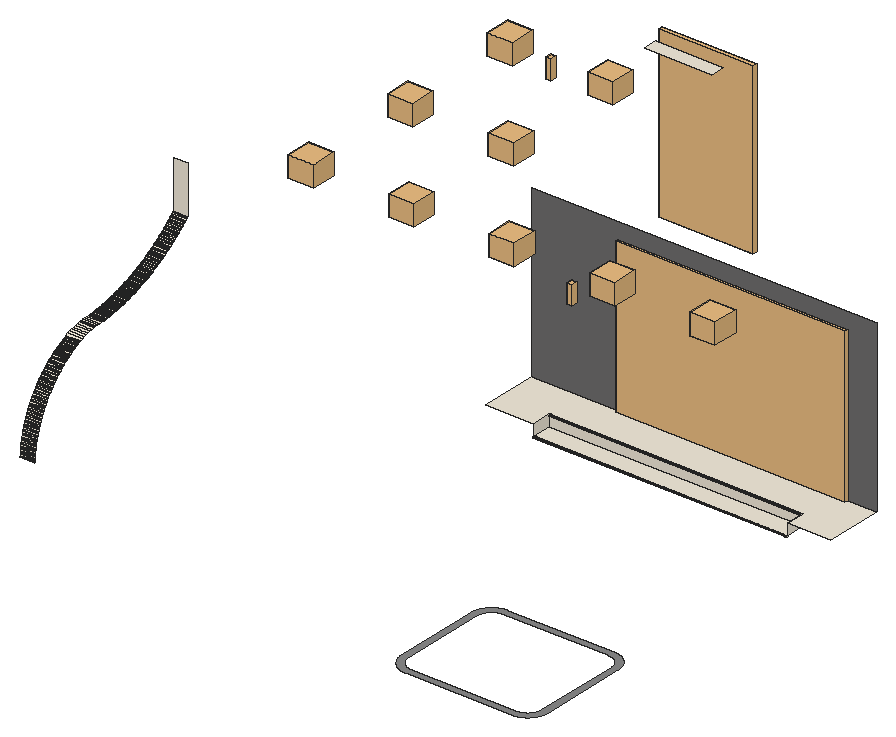
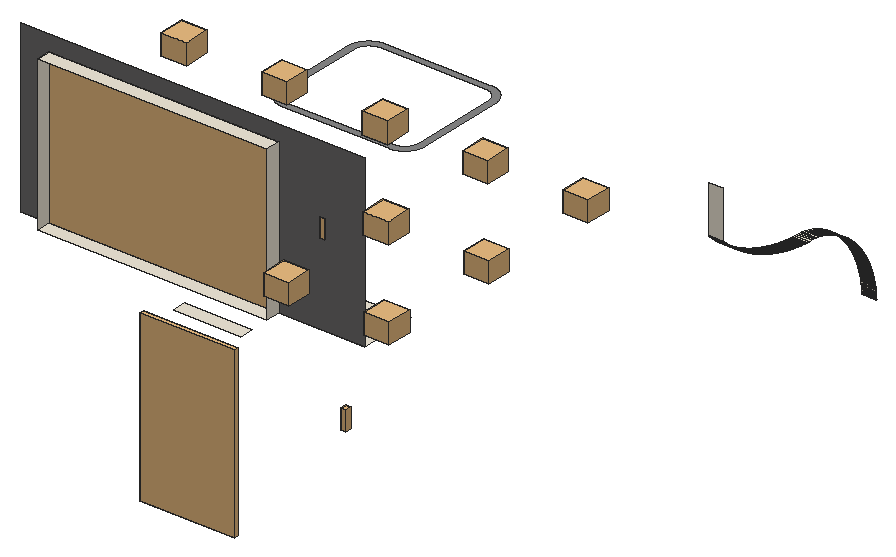
# SketchUp Ruby script. Lengths in inches.
U = 1.inch
M = Sketchup.active_model
def pt(a) = Geom::Point3d.new(a.map { |v| v * U })
def face(e, loops, mat)
  f = e.add_face(loops[0].map { |a| pt(a) })
  loops[1..].each { |l| e.add_face(l.map { |a| pt(a) }).erase! }
  f.material = f.back_material = mat if mat
  f
end
# faces: each face lists its corners as indices into pts; further lists are holes
def faces(e, pts, list, mat = nil) = list.each { |f| face(e, (f[0].is_a?(Array) ? f : [f]).map { |l| l.map { |i| pts[i] } }, mat) }
# xy, xz, yz: faces in a plane at the given z, y or x. An outline is a flat list of corners, or four numbers for a rectangle; further outlines are holes
def ring(l) = l.size == 4 ? [[l[0], l[1]], [l[2], l[1]], [l[2], l[3]], [l[0], l[3]]] : l.each_slice(2).to_a
def flat(e, list, mat, &to3) = list.each { |f| face(e, (f[0].is_a?(Array) ? f : [f]).map { |l| ring(l).map { |u, v| to3.(u, v) } }, mat) }
def xy(e, z, list, mat = nil) = flat(e, list, mat) { |x, y| [x, y, z] }
def xz(e, y, list, mat = nil) = flat(e, list, mat) { |x, z| [x, y, z] }
def yz(e, x, list, mat = nil) = flat(e, list, mat) { |y, z| [x, y, z] }
def lines(e, pts, list) = list.each { |a, b| e.add_line(pt(pts[a]), pt(pts[b])) }
# prism: a flat outline (further loops are holes) pulled along v
def prism(e, loops, v, mat = nil)
  f = face(e, loops, mat); d = Geom::Vector3d.new(v.map { |x| x * U })
  f.pushpull(f.normal.samedirection?(d) ? d.length : -d.length)
end
def box(e, o, s, mat = nil) = prism(e, [[o, [o[0] + s[0], o[1], o[2]], [o[0] + s[0], o[1] + s[1], o[2]], [o[0], o[1] + s[1], o[2]]]], [0, 0, s[2]], mat)
def at(x, y, z, deg = 0) = Geom::Transformation.translation(pt([x, y, z])) * Geom::Transformation.rotation(ORIGIN, Z_AXIS, deg.degrees)
def axes(o, x, y, z) = Geom::Transformation.new([*x, 0, *y, 0, *z, 0, *pt(o).to_a, 1])
def part(name) = M.definitions.add(name)
# library, detail: a bought-in or finely detailed component or shape, given as its bounding box
def library(name, o, s) = part(name).tap { |d| box(d.entities, o, s) }
def detail(e, o, s) = box(e.add_group.entities, o, s)
def put(e, d, t, mat = nil) = e.add_instance(d, t).tap { |i| i.material = mat if mat }
def group(e, t, mat = nil) = e.add_group.tap { |g| g.transformation = t; g.material = mat if mat }.entities
root = M.entities
M.materials.add("0027 AP L140 CRUSHED ICE").color = [241, 233, 217]
M.materials.add("[Metal Seamed]").color = [40, 40, 40]
M.materials.add("[Stone Coursed Rough]").color = [137, 137, 137]
M.materials.add("[Stone Vein Gray]").color = [112, 111, 111]
c1 = library("CURTAIN",[20.4,9.88,0],[29.77,2.88,102.36])
c2 = library("Group\#6",[0,-2,0],[144,2,96])
c3 = library("WALL LIGHT 69",[4.19,4.05,-8.78],[4.61,5.7,17.13])
c4 = library("3",[-5.94,-5.94,-13.08],[15.84,15.84,13.08])
xy(root,4,[[[291,44,357,44,357.41,44.01,357.82,44.03,358.22,44.06,358.63,44.1,359.03,44.16,359.4375,44.23,359.84,44.3125,360.23,44.41,360.625,44.52,361.02,44.64,361.4,44.77,361.79,44.91,362.16,45.07,362.54,45.24,362.9,45.42,363.26,45.61,363.62,45.81,363.97,46.02,364.31,46.25,364.64,46.48,364.97,46.73,365.29,46.98,365.6,47.25,365.9,47.52,366.48,48.1,366.75,48.4,367.02,48.71,367.27,49.03,367.52,49.36,367.75,49.69,367.98,50.03,368.19,50.38,368.39,50.74,368.58,51.1,368.76,51.46,368.93,51.84,369.09,52.21,369.23,52.6,369.36,52.98,369.48,53.375,369.59,53.77,369.6875,54.16,369.77,54.5625,369.84,54.97,369.9,55.37,369.94,55.78,369.97,56.18,369.99,56.59,370,57,370,111,369.99,111.41,369.97,111.82,369.94,112.22,369.9,112.63,369.84,113.03,369.77,113.4375,369.6875,113.84,369.59,114.23,369.48,114.625,369.36,115.02,369.23,115.4,369.09,115.79,368.93,116.16,368.76,116.54,368.58,116.9,368.39,117.26,368.19,117.62,367.98,117.97,367.75,118.31,367.52,118.64,367.27,118.97,367.02,119.29,366.75,119.6,366.48,119.9,365.9,120.48,365.6,120.75,365.29,121.02,364.97,121.27,364.64,121.52,364.31,121.75,363.97,121.98,363.62,122.19,363.26,122.39,362.9,122.58,362.54,122.76,362.16,122.93,361.79,123.09,361.4,123.23,361.02,123.36,360.625,123.48,360.23,123.59,359.84,123.6875,359.4375,123.77,359.03,123.84,358.63,123.9,358.22,123.94,357.82,123.97,357.41,123.99,357,124,291,124,290.59,123.99,290.18,123.97,289.78,123.94,289.37,123.9,288.97,123.84,288.5625,123.77,288.16,123.6875,287.77,123.59,287.375,123.48,286.98,123.36,286.6,123.23,286.21,123.09,285.84,122.93,285.46,122.76,285.1,122.58,284.74,122.39,284.38,122.19,284.03,121.98,283.69,121.75,283.36,121.52,283.03,121.27,282.71,121.02,282.4,120.75,282.1,120.48,281.52,119.9,281.25,119.6,280.98,119.29,280.73,118.97,280.48,118.64,280.25,118.31,280.02,117.97,279.81,117.62,279.61,117.26,279.42,116.9,279.24,116.54,279.07,116.16,278.91,115.79,278.77,115.4,278.64,115.02,278.52,114.625,278.41,114.23,278.3125,113.84,278.23,113.4375,278.16,113.03,278.1,112.63,278.06,112.22,278.03,111.82,278.01,111.41,278,111,278,57,278.01,56.59,278.03,56.18,278.06,55.78,278.1,55.37,278.16,54.97,278.23,54.5625,278.3125,54.16,278.41,53.77,278.52,53.375,278.64,52.98,278.77,52.6,278.91,52.21,279.07,51.84,279.24,51.46,279.42,51.1,279.61,50.74,279.81,50.38,280.02,50.03,280.25,49.69,280.48,49.36,280.73,49.03,280.98,48.71,281.25,48.4,281.52,48.1,282.1,47.52,282.4,47.25,282.71,46.98,283.03,46.73,283.36,46.48,283.69,46.25,284.03,46.02,284.38,45.81,284.74,45.61,285.1,45.42,285.46,45.24,285.84,45.07,286.21,44.91,286.6,44.77,286.98,44.64,287.375,44.52,287.77,44.41,288.16,44.3125,288.5625,44.23,288.97,44.16,289.37,44.1,289.78,44.06,290.18,44.03,290.59,44.01],[290.72,48,290.43,48.02,290.15,48.04,289.87,48.07,289.59,48.11,289.3125,48.16,289.04,48.22,288.76,48.28,288.22,48.44,287.95,48.53,287.6875,48.63,287.43,48.74,286.91,48.98,286.66,49.11,286.42,49.25,286.18,49.4,285.94,49.56,285.71,49.72,285.48,49.89,285.26,50.07,285.05,50.25,284.84,50.4375,284.64,50.64,284.4375,50.84,284.25,51.05,284.07,51.26,283.89,51.48,283.72,51.71,283.56,51.94,283.4,52.18,283.25,52.42,283.11,52.66,282.98,52.91,282.74,53.43,282.63,53.6875,282.53,53.95,282.44,54.22,282.28,54.76,282.22,55.04,282.16,55.3125,282.11,55.59,282.07,55.87,282.04,56.15,282.02,56.43,282,56.72,282,111.28,282.02,111.57,282.04,111.85,282.07,112.13,282.11,112.41,282.16,112.6875,282.22,112.96,282.28,113.24,282.44,113.78,282.53,114.05,282.63,114.3125,282.74,114.57,282.98,115.09,283.11,115.34,283.25,115.58,283.4,115.82,283.56,116.06,283.72,116.29,283.89,116.52,284.07,116.74,284.25,116.95,284.4375,117.16,284.64,117.36,284.84,117.5625,285.05,117.75,285.26,117.93,285.48,118.11,285.71,118.28,285.94,118.44,286.18,118.6,286.42,118.75,286.66,118.89,286.91,119.02,287.43,119.26,287.6875,119.37,287.95,119.47,288.22,119.56,288.76,119.72,289.04,119.78,289.3125,119.84,289.59,119.89,289.87,119.93,290.15,119.96,290.43,119.98,290.72,120,357.28,120,357.57,119.98,357.85,119.96,358.13,119.93,358.41,119.89,358.6875,119.84,358.96,119.78,359.24,119.72,359.78,119.56,360.05,119.47,360.3125,119.37,360.57,119.26,361.09,119.02,361.34,118.89,361.58,118.75,361.82,118.6,362.06,118.44,362.29,118.28,362.52,118.11,362.74,117.93,362.95,117.75,363.16,117.5625,363.36,117.36,363.5625,117.16,363.75,116.95,363.93,116.74,364.11,116.52,364.28,116.29,364.44,116.06,364.6,115.82,364.75,115.58,364.89,115.34,365.02,115.09,365.26,114.57,365.37,114.3125,365.47,114.05,365.56,113.78,365.72,113.24,365.78,112.96,365.84,112.6875,365.89,112.41,365.93,112.13,365.96,111.85,365.98,111.57,366,111.28,366,56.72,365.98,56.43,365.96,56.15,365.93,55.87,365.89,55.59,365.84,55.3125,365.78,55.04,365.72,54.76,365.56,54.22,365.47,53.95,365.37,53.6875,365.26,53.43,365.02,52.91,364.89,52.66,364.75,52.42,364.6,52.18,364.44,51.94,364.28,51.71,364.11,51.48,363.93,51.26,363.75,51.05,363.5625,50.84,363.36,50.64,363.16,50.4375,362.95,50.25,362.74,50.07,362.52,49.89,362.29,49.72,362.06,49.56,361.82,49.4,361.58,49.25,361.34,49.11,361.09,48.98,360.57,48.74,360.3125,48.63,360.05,48.53,359.78,48.44,359.24,48.28,358.96,48.22,358.6875,48.16,358.41,48.11,358.13,48.07,357.85,48.04,357.57,48.02,357.28,48]]],"[Stone Coursed Rough]")
xy(root,6,[[195,263.96,354,264]],"0027 AP L140 CRUSHED ICE")
xy(root,6.01,[[195,263.88,354,263.92]],"0027 AP L140 CRUSHED ICE")
xy(root,6.99,[[195,263.88,354,263.92]],"0027 AP L140 CRUSHED ICE")
xy(root,7,[[195,263.96,354,264],[195,264,354,276]],"0027 AP L140 CRUSHED ICE")
xy(root,13,[[195,275.96,354,276]],"0027 AP L140 CRUSHED ICE")
xy(root,13.01,[[195,275.88,354,275.92]],"0027 AP L140 CRUSHED ICE")
xy(root,13.99,[[195,275.88,354,275.92]],"0027 AP L140 CRUSHED ICE")
xy(root,14,[[165,264,195,264,195,276,354,276,354,264,381,264,381,300,363,300,363,309,219,309,219,300,165,300],[195,275.96,354,276]],"0027 AP L140 CRUSHED ICE")
xy(root,110,[[219,300,363,309]],"0027 AP L140 CRUSHED ICE")
xy(root,111,[[111,456,153,465]],"0027 AP L140 CRUSHED ICE")
xz(root,214,[[9,90,18,120]],"0027 AP L140 CRUSHED ICE")
xz(root,263.5,[[195,6.46,354,6.5],[195,6.5,354,6.54]],"0027 AP L140 CRUSHED ICE")
xz(root,263.51,[[195,6.38,354,6.42],[195,6.58,354,6.62]],"0027 AP L140 CRUSHED ICE")
xz(root,275.5,[[195,13.46,354,13.5],[195,13.5,354,13.54]],"0027 AP L140 CRUSHED ICE")
xz(root,275.51,[[195,13.38,354,13.42],[195,13.58,354,13.62]],"0027 AP L140 CRUSHED ICE")
xz(root,276,[[195,7,354,13]],"0027 AP L140 CRUSHED ICE")
xz(root,300,[[165,14,219,14,219,110,363,110,363,14,381,14,381,120,165,120]],"[Stone Vein Gray]")
yz(root,195,[[263.96,6,263.92,6.01,263.88,6.01,263.85,6.02,263.81,6.04,263.77,6.05,263.74,6.07,263.71,6.1,263.68,6.12,263.62,6.18,263.6,6.21,263.57,6.24,263.55,6.27,263.54,6.31,263.52,6.35,263.51,6.38,263.51,6.42,263.5,6.46,263.5,6.54,263.51,6.58,263.51,6.62,263.52,6.65,263.54,6.69,263.55,6.73,263.57,6.76,263.6,6.79,263.62,6.82,263.68,6.88,263.71,6.9,263.74,6.93,263.77,6.95,263.81,6.96,263.85,6.98,263.88,6.99,263.92,6.99,263.96,7,264,7,264,6],[264,7,276,7,276,13,275.96,13,275.92,13.01,275.88,13.01,275.85,13.02,275.81,13.04,275.77,13.05,275.74,13.07,275.71,13.1,275.68,13.12,275.62,13.18,275.6,13.21,275.57,13.24,275.55,13.27,275.54,13.31,275.52,13.35,275.51,13.38,275.51,13.42,275.5,13.46,275.5,13.54,275.51,13.58,275.51,13.62,275.52,13.65,275.54,13.69,275.55,13.73,275.57,13.76,275.6,13.79,275.62,13.82,275.68,13.88,275.71,13.9,275.74,13.93,275.77,13.95,275.81,13.96,275.85,13.98,275.88,13.99,275.92,13.99,275.96,14,276,14,264,14],[275.96,13,276,13,276,14,275.96,14,275.92,13.99,275.88,13.99,275.85,13.98,275.81,13.96,275.77,13.95,275.74,13.93,275.71,13.9,275.68,13.88,275.62,13.82,275.6,13.79,275.57,13.76,275.55,13.73,275.54,13.69,275.52,13.65,275.51,13.62,275.51,13.58,275.5,13.54,275.5,13.46,275.51,13.42,275.51,13.38,275.52,13.35,275.54,13.31,275.55,13.27,275.57,13.24,275.6,13.21,275.62,13.18,275.68,13.12,275.71,13.1,275.74,13.07,275.77,13.05,275.81,13.04,275.85,13.02,275.88,13.01,275.92,13.01]],"0027 AP L140 CRUSHED ICE")
yz(root,219,[[300,14,309,110]],"0027 AP L140 CRUSHED ICE")
yz(root,354,[[263.96,6,264,6,264,7,263.96,7,263.92,6.99,263.88,6.99,263.85,6.98,263.81,6.96,263.77,6.95,263.74,6.93,263.71,6.9,263.68,6.88,263.62,6.82,263.6,6.79,263.57,6.76,263.55,6.73,263.54,6.69,263.52,6.65,263.51,6.62,263.51,6.58,263.5,6.54,263.5,6.46,263.51,6.42,263.51,6.38,263.52,6.35,263.54,6.31,263.55,6.27,263.57,6.24,263.6,6.21,263.62,6.18,263.68,6.12,263.71,6.1,263.74,6.07,263.77,6.05,263.81,6.04,263.85,6.02,263.88,6.01,263.92,6.01],[264,7,264,14,276,14,275.96,14,275.92,13.99,275.88,13.99,275.85,13.98,275.81,13.96,275.77,13.95,275.74,13.93,275.71,13.9,275.68,13.88,275.62,13.82,275.6,13.79,275.57,13.76,275.55,13.73,275.54,13.69,275.52,13.65,275.51,13.62,275.51,13.58,275.5,13.54,275.5,13.46,275.51,13.42,275.51,13.38,275.52,13.35,275.54,13.31,275.55,13.27,275.57,13.24,275.6,13.21,275.62,13.18,275.68,13.12,275.71,13.1,275.74,13.07,275.77,13.05,275.81,13.04,275.85,13.02,275.88,13.01,275.92,13.01,275.96,13,276,13,276,7],[275.96,13,275.92,13.01,275.88,13.01,275.85,13.02,275.81,13.04,275.77,13.05,275.74,13.07,275.71,13.1,275.68,13.12,275.62,13.18,275.6,13.21,275.57,13.24,275.55,13.27,275.54,13.31,275.52,13.35,275.51,13.38,275.51,13.42,275.5,13.46,275.5,13.54,275.51,13.58,275.51,13.62,275.52,13.65,275.54,13.69,275.55,13.73,275.57,13.76,275.6,13.79,275.62,13.82,275.68,13.88,275.71,13.9,275.74,13.93,275.77,13.95,275.81,13.96,275.85,13.98,275.88,13.99,275.92,13.99,275.96,14,276,14,276,13]],"0027 AP L140 CRUSHED ICE")
yz(root,363,[[300,14,309,110]],"0027 AP L140 CRUSHED ICE")
p = [[18,94,4.5],[18,94.01,4.73],[9,94.01,4.73],[9,94,4.5],[18,94.04,5.41],[9,94.04,5.41],
  [18,94.08,6.08],[9,94.08,6.08],[354,263.88,6.01],[354,263.85,6.02],[195,263.85,6.02],[195,263.88,6.01],
  [354,263.81,6.04],[195,263.81,6.04],[354,263.77,6.05],[195,263.77,6.05],[354,263.96,6],[354,263.92,6.01],
  [195,263.92,6.01],[195,263.96,6],[18,94.13,6.76],[9,94.13,6.76],[354,263.68,6.12],[354,263.65,6.15],
  [195,263.65,6.15],[195,263.68,6.12],[354,263.62,6.18],[195,263.62,6.18],[354,263.74,6.07],[195,263.74,6.07],
  [354,263.71,6.1],[195,263.71,6.1],[354,263.6,6.21],[195,263.6,6.21],[354,263.57,6.24],[195,263.57,6.24],
  [354,263.55,6.27],[195,263.55,6.27],[354,263.54,6.31],[195,263.54,6.31],[354,263.52,6.35],[195,263.52,6.35],
  [354,263.51,6.38],[195,263.51,6.38],[354,263.51,6.42],[354,263.5,6.46],[195,263.5,6.46],[195,263.51,6.42],
  [354,263.5,6.54],[354,263.51,6.58],[195,263.51,6.58],[195,263.5,6.54],[354,263.51,6.62],[354,263.52,6.65],
  [195,263.52,6.65],[195,263.51,6.62],[354,263.54,6.69],[195,263.54,6.69],[354,263.55,6.73],[195,263.55,6.73],
  [354,263.57,6.76],[195,263.57,6.76],[18,94.18,7.43],[9,94.18,7.43],[354,263.6,6.79],[195,263.6,6.79],
  [354,263.62,6.82],[195,263.62,6.82],[354,263.65,6.85],[195,263.65,6.85],[354,263.68,6.88],[195,263.68,6.88],
  [354,263.71,6.9],[195,263.71,6.9],[354,263.74,6.93],[195,263.74,6.93],[354,263.77,6.95],[195,263.77,6.95],
  [354,263.81,6.96],[195,263.81,6.96],[354,263.85,6.98],[195,263.85,6.98],[354,263.88,6.99],[195,263.88,6.99],
  [354,263.92,6.99],[354,263.96,7],[195,263.96,7],[195,263.92,6.99],[18,94.24,8.1],[9,94.24,8.1],
  [18,94.31,8.78],[9,94.31,8.78],[18,94.39,9.45],[9,94.39,9.45],[18,94.48,10.12],[9,94.48,10.12],
  [18,94.57,10.79],[9,94.57,10.79],[18,94.67,11.46],[9,94.67,11.46],[18,94.78,12.125],[9,94.78,12.125],
  [18,94.9,12.79],[9,94.9,12.79],[18,95.02,13.45],[9,95.02,13.45],[354,275.88,13.01],[354,275.85,13.02],
  [195,275.85,13.02],[195,275.88,13.01],[354,275.81,13.04],[195,275.81,13.04],[354,275.77,13.05],[195,275.77,13.05],
  [354,275.96,13],[354,275.92,13.01],[195,275.92,13.01],[195,275.96,13],[354,275.68,13.12],[354,275.65,13.15],
  [195,275.65,13.15],[195,275.68,13.12],[354,275.62,13.18],[195,275.62,13.18],[354,275.74,13.07],[195,275.74,13.07],
  [354,275.71,13.1],[195,275.71,13.1],[354,275.6,13.21],[195,275.6,13.21],[354,275.57,13.24],[195,275.57,13.24],
  [354,275.55,13.27],[195,275.55,13.27],[354,275.54,13.31],[195,275.54,13.31],[354,275.52,13.35],[195,275.52,13.35],
  [354,275.51,13.38],[195,275.51,13.38],[354,275.51,13.42],[354,275.5,13.46],[195,275.5,13.46],[195,275.51,13.42],
  [18,95.15,14.12],[9,95.15,14.12],[354,275.5,13.54],[354,275.51,13.58],[195,275.51,13.58],[195,275.5,13.54],
  [354,275.51,13.62],[354,275.52,13.65],[195,275.52,13.65],[195,275.51,13.62],[354,275.54,13.69],[195,275.54,13.69],
  [354,275.55,13.73],[195,275.55,13.73],[354,275.57,13.76],[195,275.57,13.76],[354,275.6,13.79],[195,275.6,13.79],
  [354,275.62,13.82],[195,275.62,13.82],[354,275.65,13.85],[195,275.65,13.85],[354,275.68,13.88],[195,275.68,13.88],
  [354,275.71,13.9],[195,275.71,13.9],[354,275.74,13.93],[195,275.74,13.93],[354,275.77,13.95],[195,275.77,13.95],
  [354,275.81,13.96],[195,275.81,13.96],[354,275.85,13.98],[195,275.85,13.98],[354,275.88,13.99],[195,275.88,13.99],
  [354,275.92,13.99],[354,275.96,14],[195,275.96,14],[195,275.92,13.99],[18,95.29,14.78],[9,95.29,14.78],
  [18,95.43,15.44],[9,95.43,15.44],[18,95.59,16.1],[9,95.59,16.1],[18,95.75,16.76],[9,95.75,16.76],
  [18,95.92,17.41],[9,95.92,17.41],[18,96.08,18],[18,96.09,18.0625],[9,96.09,18.0625],[18,96.28,18.71],
  [9,96.28,18.71],[18,96.47,19.36],[9,96.47,19.36],[18,96.66,20.01],[9,96.66,20.01],[18,96.87,20.65],
  [9,96.87,20.65],[18,97.08,21.3],[9,97.08,21.3],[18,97.3,21.93],[9,97.3,21.93],[18,97.53,22.57],
  [9,97.53,22.57],[18,97.76,23.21],[9,97.76,23.21],[18,98.01,23.84],[9,98.01,23.84],[18,98.25,24.47],
  [9,98.25,24.47],[18,98.51,25.09],[9,98.51,25.09],[18,98.77,25.71],[9,98.77,25.71],[18,99.04,26.33],
  [9,99.04,26.33],[18,99.32,26.95],[9,99.32,26.95],[18,99.6,27.57],[9,99.6,27.57],[18,99.89,28.18],
  [9,99.89,28.18],[18,100.19,28.78],[9,100.19,28.78],[18,100.5,29.39],[9,100.5,29.39],[18,100.81,29.99],
  [9,100.81,29.99],[18,101.125,30.58],[9,101.125,30.58],[18,101.45,31.18],[9,101.45,31.18],[18,101.78,31.76],
  [9,101.78,31.76],[18,102.12,32.35],[9,102.12,32.35],[18,102.47,32.93],[9,102.47,32.93],[18,102.82,33.51],
  [9,102.82,33.51],[18,103.18,34.08],[9,103.18,34.08],[18,103.54,34.65],[9,103.54,34.65],[18,103.91,35.22],
  [9,103.91,35.22],[18,104.29,35.78],[9,104.29,35.78],[18,104.67,36.33],[9,104.67,36.33],[18,105.0625,36.89],
  [9,105.0625,36.89],[18,105.46,37.43],[9,105.46,37.43],[18,105.86,37.98],[9,105.86,37.98],[18,106.27,38.52],
  [9,106.27,38.52],[18,106.6875,39.05],[9,106.6875,39.05],[18,107.11,39.58],[9,107.11,39.58],[18,107.53,40.1],
  [9,107.53,40.1],[18,107.97,40.625],[9,107.97,40.625],[18,108.41,41.14],[9,108.41,41.14],[18,108.85,41.65],
  [9,108.85,41.65],[18,109.3,42.15],[9,109.3,42.15],[18,109.76,42.65],[9,109.76,42.65],[18,110.22,43.14],
  [9,110.22,43.14],[18,110.69,43.63],[9,110.69,43.63],[18,111.16,44.12],[9,111.16,44.12],[18,111.64,44.6],
  [9,111.64,44.6],[18,112.12,45.07],[9,112.12,45.07],[18,112.61,45.53],[9,112.61,45.53],[18,113.1,46],
  [9,113.1,46],[18,113.6,46.45],[9,113.6,46.45],[18,114.11,46.9],[9,114.11,46.9],[18,114.62,47.35],
  [9,114.62,47.35],[18,115.13,47.79],[9,115.13,47.79],[18,115.65,48.22],[9,115.65,48.22],[18,116.17,48.64],
  [9,116.17,48.64],[18,116.7,49.07],[9,116.7,49.07],[18,117.24,49.48],[9,117.24,49.48],[18,117.78,49.89],
  [9,117.78,49.89],[18,118.32,50.29],[9,118.32,50.29],[18,118.87,50.6875],[9,118.87,50.6875],[18,119.42,51.08],
  [9,119.42,51.08],[18,119.98,51.46],[9,119.98,51.46],[18,120.54,51.84],[9,120.54,51.84],[18,121.1,52.21],
  [9,121.1,52.21],[18,121.67,52.57],[9,121.67,52.57],[18,122.25,52.93],[9,122.25,52.93],[18,122.82,53.28],
  [9,122.82,53.28],[18,123.4,53.63],[9,123.4,53.63],[18,123.99,53.97],[9,123.99,53.97],[18,124.58,54.3],
  [9,124.58,54.3],[18,125.17,54.625],[9,125.17,54.625],[18,125.77,54.94],[9,125.77,54.94],[18,126.37,55.25],
  [9,126.37,55.25],[18,126.97,55.56],[9,126.97,55.56],[18,127.58,55.86],[9,127.58,55.86],[18,128.19,56.15],
  [9,128.19,56.15],[18,128.8,56.43],[9,128.8,56.43],[18,129.42,56.71],[9,129.42,56.71],[18,130.04,56.98],
  [9,130.04,56.98],[18,131.46,57.56],[9,131.46,57.56],[18,132.9,58.08],[9,132.9,58.08],[18,134.35,58.55],
  [9,134.35,58.55],[18,135.83,58.98],[9,135.83,58.98],[18,137.3125,59.34],[9,137.3125,59.34],[18,138.8125,59.65],
  [9,138.8125,59.65],[18,140.32,59.91],[9,140.32,59.91],[18,141.15,60.02],[9,141.15,60.02],[18,141.84,60.12],
  [9,141.84,60.12],[18,143.36,60.27],[9,143.36,60.27],[18,144.89,60.36],[9,144.89,60.36],[18,146.42,60.4],
  [9,146.42,60.4],[18,147.95,60.38],[9,147.95,60.38],[18,148.64,60.4375],[9,148.64,60.4375],[18,149.33,60.5],
  [9,149.33,60.5],[18,150.01,60.57],[9,150.01,60.57],[18,150.7,60.64],[9,150.7,60.64],[18,151.38,60.72],
  [9,151.38,60.72],[18,152.07,60.8],[9,152.07,60.8],[18,152.75,60.89],[9,152.75,60.89],[18,153.4375,60.98],
  [9,153.4375,60.98],[18,154.12,61.07],[9,154.12,61.07],[18,154.8,61.17],[9,154.8,61.17],[18,155.48,61.27],
  [9,155.48,61.27],[18,156.17,61.38],[9,156.17,61.38],[18,156.85,61.49],[9,156.85,61.49],[18,157.53,61.61],
  [9,157.53,61.61],[18,158.21,61.73],[9,158.21,61.73],[18,158.88,61.85],[9,158.88,61.85],[18,159.5625,61.98],
  [9,159.5625,61.98],[18,160.24,62.11],[9,160.24,62.11],[18,160.91,62.25],[9,160.91,62.25],[18,161.59,62.39],
  [9,161.59,62.39],[18,162.26,62.54],[9,162.26,62.54],[18,162.94,62.6875],[9,162.94,62.6875],[18,163.61,62.84],
  [9,163.61,62.84],[18,164.28,63],[9,164.28,63],[18,164.95,63.16],[9,164.95,63.16],[18,165.62,63.33],
  [9,165.62,63.33],[18,166.29,63.5],[9,166.29,63.5],[18,166.95,63.68],[9,166.95,63.68],[18,167.62,63.86],
  [9,167.62,63.86],[18,168.28,64.04],[9,168.28,64.04],[18,168.95,64.23],[9,168.95,64.23],[18,169.61,64.42],
  [9,169.61,64.42],[18,170.27,64.62],[9,170.27,64.62],[18,170.93,64.82],[9,170.93,64.82],[18,171.59,65.02],
  [9,171.59,65.02],[18,172.24,65.23],[9,172.24,65.23],[18,172.9,65.44],[9,172.9,65.44],[18,173.55,65.66],
  [9,173.55,65.66],[18,174.21,65.88],[9,174.21,65.88],[18,174.86,66.11],[9,174.86,66.11],[18,175.51,66.34],
  [9,175.51,66.34],[18,176.16,66.57],[9,176.16,66.57],[18,176.81,66.81],[9,176.81,66.81],[18,177.45,67.05],
  [9,177.45,67.05],[18,178.1,67.3],[9,178.1,67.3],[18,178.74,67.55],[9,178.74,67.55],[18,179.38,67.8],
  [9,179.38,67.8],[18,180.02,68.06],[9,180.02,68.06],[18,180.66,68.32],[9,180.66,68.32],[18,181.29,68.59],
  [9,181.29,68.59],[18,181.93,68.86],[9,181.93,68.86],[18,182.56,69.13],[9,182.56,69.13],[18,183.19,69.41],
  [9,183.19,69.41],[18,183.82,69.69],[9,183.82,69.69],[18,184.45,69.98],[9,184.45,69.98],[18,185.07,70.27],
  [9,185.07,70.27],[18,185.7,70.5625],[9,185.7,70.5625],[18,186.32,70.86],[9,186.32,70.86],[18,186.9375,71.16],
  [9,186.9375,71.16],[18,187.56,71.47],[9,187.56,71.47],[18,188.17,71.78],[9,188.17,71.78],[18,188.79,72.09],
  [9,188.79,72.09],[18,189.4,72.41],[9,189.4,72.41],[18,190.01,72.73],[9,190.01,72.73],[18,190.62,73.06],
  [9,190.62,73.06],[18,191.22,73.38],[9,191.22,73.38],[18,191.83,73.72],[9,191.83,73.72],[18,192.43,74.05],
  [9,192.43,74.05],[18,193.03,74.39],[9,193.03,74.39],[18,193.625,74.74],[9,193.625,74.74],[18,194.22,75.09],
  [9,194.22,75.09],[18,194.8125,75.4375],[9,194.8125,75.4375],[18,195.41,75.79],[9,195.41,75.79],[18,195.99,76.15],
  [9,195.99,76.15],[18,196.58,76.52],[9,196.58,76.52],[18,197.16,76.88],[9,197.16,76.88],[18,197.75,77.25],
  [9,197.75,77.25],[18,198.32,77.63],[9,198.32,77.63],[18,198.9,78.01],[9,198.9,78.01],[18,199.48,78.39],
  [9,199.48,78.39],[18,200.05,78.77],[9,200.05,78.77],[18,200.62,79.16],[9,200.62,79.16],[18,201.19,79.55],
  [9,201.19,79.55],[18,201.75,79.95],[9,201.75,79.95],[18,202.3125,80.35],[9,202.3125,80.35],[18,202.87,80.75],
  [9,202.87,80.75],[18,203.43,81.16],[9,203.43,81.16],[18,203.98,81.57],[9,203.98,81.57],[18,204.54,81.98],
  [9,204.54,81.98],[18,205.08,82.4],[9,205.08,82.4],[18,205.63,82.82],[9,205.63,82.82],[18,206.18,83.24],
  [9,206.18,83.24],[18,206.72,83.67],[9,206.72,83.67],[18,207.26,84.1],[9,207.26,84.1],[18,207.79,84.53],
  [9,207.79,84.53],[18,208.32,84.97],[9,208.32,84.97],[18,208.85,85.41],[9,208.85,85.41],[18,209.38,85.86],
  [9,209.38,85.86],[18,209.91,86.3],[9,209.91,86.3],[18,210.43,86.75],[9,210.43,86.75],[18,210.95,87.21],
  [9,210.95,87.21],[18,211.46,87.67],[9,211.46,87.67],[18,211.98,88.125],[9,211.98,88.125],[18,212.49,88.59],
  [9,212.49,88.59],[18,212.99,89.06],[9,212.99,89.06],[18,213.5,89.53],[9,213.5,89.53],[18,214,90],
  [9,214,90],[18,95.92,18]]
faces(root,p,[[0,1,2,3],[1,4,5,2],[4,6,7,5],[8,9,10,11],[9,12,13,10],[12,14,15,13],[16,17,18,19],[6,20,21,7],
  [22,23,24,25],[23,26,27,24],[14,28,29,15],[28,30,31,29],[30,22,25,31],[26,32,33,27],[32,34,35,33],[34,36,37,35],
  [36,38,39,37],[38,40,41,39],[40,42,43,41],[44,45,46,47],[48,49,50,51],[52,53,54,55],[53,56,57,54],[56,58,59,57],
  [58,60,61,59],[20,62,63,21],[60,64,65,61],[64,66,67,65],[66,68,69,67],[68,70,71,69],[70,72,73,71],[72,74,75,73],
  [74,76,77,75],[76,78,79,77],[78,80,81,79],[80,82,83,81],[84,85,86,87],[62,88,89,63],[88,90,91,89],[90,92,93,91],
  [92,94,95,93],[94,96,97,95],[96,98,99,97],[98,100,101,99],[100,102,103,101],[102,104,105,103],[106,107,108,109],[107,110,111,108],
  [110,112,113,111],[114,115,116,117],[118,119,120,121],[119,122,123,120],[112,124,125,113],[124,126,127,125],[126,118,121,127],[122,128,129,123],
  [128,130,131,129],[130,132,133,131],[132,134,135,133],[134,136,137,135],[136,138,139,137],[140,141,142,143],[104,144,145,105],[146,147,148,149],
  [150,151,152,153],[151,154,155,152],[154,156,157,155],[156,158,159,157],[158,160,161,159],[160,162,163,161],[162,164,165,163],[164,166,167,165],
  [166,168,169,167],[168,170,171,169],[170,172,173,171],[172,174,175,173],[174,176,177,175],[176,178,179,177],[180,181,182,183],[144,184,185,145],
  [184,186,187,185],[186,188,189,187],[188,190,191,189],[190,192,193,191],[194,195,196,193,192],[195,197,198,196],[197,199,200,198],[199,201,202,200],
  [201,203,204,202],[203,205,206,204],[205,207,208,206],[207,209,210,208],[209,211,212,210],[211,213,214,212],[213,215,216,214],[215,217,218,216],
  [217,219,220,218],[219,221,222,220],[221,223,224,222],[223,225,226,224],[225,227,228,226],[227,229,230,228],[229,231,232,230],[231,233,234,232],
  [233,235,236,234],[235,237,238,236],[237,239,240,238],[239,241,242,240],[241,243,244,242],[243,245,246,244],[245,247,248,246],[247,249,250,248],
  [249,251,252,250],[251,253,254,252],[253,255,256,254],[255,257,258,256],[257,259,260,258],[259,261,262,260],[261,263,264,262],[263,265,266,264],
  [265,267,268,266],[267,269,270,268],[269,271,272,270],[271,273,274,272],[273,275,276,274],[275,277,278,276],[277,279,280,278],[279,281,282,280],
  [281,283,284,282],[283,285,286,284],[285,287,288,286],[287,289,290,288],[289,291,292,290],[291,293,294,292],[293,295,296,294],[295,297,298,296],
  [297,299,300,298],[299,301,302,300],[301,303,304,302],[303,305,306,304],[305,307,308,306],[307,309,310,308],[309,311,312,310],[311,313,314,312],
  [313,315,316,314],[315,317,318,316],[317,319,320,318],[319,321,322,320],[321,323,324,322],[323,325,326,324],[325,327,328,326],[327,329,330,328],
  [329,331,332,330],[331,333,334,332],[333,335,336,334],[335,337,338,336],[337,339,340,338],[339,341,342,340],[341,343,344,342],[343,345,346,344],
  [345,347,348,346],[347,349,350,348],[349,351,352,350],[351,353,354,352],[353,355,356,354],[355,357,358,356],[357,359,360,358],[359,361,362,360],
  [361,363,364,362],[363,365,366,364],[365,367,368,366],[367,369,370,368],[369,371,372,370],[371,373,374,372],[373,375,376,374],[375,377,378,376],
  [377,379,380,378],[379,381,382,380],[381,383,384,382],[383,385,386,384],[385,387,388,386],[387,389,390,388],[389,391,392,390],[391,393,394,392],
  [393,395,396,394],[395,397,398,396],[397,399,400,398],[399,401,402,400],[401,403,404,402],[403,405,406,404],[405,407,408,406],[407,409,410,408],
  [409,411,412,410],[411,413,414,412],[413,415,416,414],[415,417,418,416],[417,419,420,418],[419,421,422,420],[421,423,424,422],[423,425,426,424],
  [425,427,428,426],[427,429,430,428],[429,431,432,430],[431,433,434,432],[433,435,436,434],[435,437,438,436],[437,439,440,438],[439,441,442,440],
  [441,443,444,442],[443,445,446,444],[445,447,448,446],[447,449,450,448],[449,451,452,450],[451,453,454,452],[453,455,456,454],[455,457,458,456],
  [457,459,460,458],[459,461,462,460],[461,463,464,462],[463,465,466,464],[465,467,468,466],[467,469,470,468],[469,471,472,470],[471,473,474,472],
  [473,475,476,474],[475,477,478,476],[477,479,480,478],[479,481,482,480],[481,483,484,482],[483,485,486,484],[485,487,488,486],[487,489,490,488],
  [489,491,492,490],[491,493,494,492],[493,495,496,494],[495,497,498,496],[497,499,500,498],[499,501,502,500],[501,503,504,502],[503,505,506,504],
  [505,507,508,506],[507,509,510,508],[509,511,512,510],[511,513,514,512],[513,515,516,514],[515,517,518,516],[517,519,520,518],[519,521,522,520],
  [521,523,524,522],[523,525,526,524],[525,527,528,526],[527,529,530,528],[529,531,532,530],[531,533,534,532],[533,535,536,534],[535,537,538,536],
  [537,539,540,538],[539,541,542,540],[541,543,544,542],[543,545,546,544],[545,547,548,546],[547,549,550,548],[549,551,552,550],[551,553,554,552],
  [553,555,556,554],[555,557,558,556],[557,559,560,558],[559,561,562,560],[561,563,564,562],[563,565,566,564],[565,567,568,566],[567,569,570,568],
  [569,571,572,570],[571,573,574,572],[573,575,576,574],[575,577,578,576],[577,579,580,578],[579,581,582,580],[581,583,584,582],[583,585,586,584],
  [585,587,588,586],[587,589,590,588],[589,591,592,590],[591,593,594,592]],"0027 AP L140 CRUSHED ICE")
lines(root,p,[[194,595]])
put(root,c1,axes([63.62,465,5.93],[2,0,0],[0,1,0],[0,0,1.03]))
put(root,c2,at(219,300,14),"[Metal Seamed]")
put(root,c3,axes([186.97,293.18,71.36],[0.7,0,0],[0,0.7,0],[0,0,0.7]),"0027 AP L140 CRUSHED ICE")
put(root,c3,axes([48.72,449.68,80.85],[0.7,0,0],[0,0.7,0],[0,0,0.7]),"0027 AP L140 CRUSHED ICE")
put(root,c4,at(184.02,256.02,121.01),"0027 AP L140 CRUSHED ICE")
put(root,c4,at(247.02,256.02,121.01),"0027 AP L140 CRUSHED ICE")
put(root,c4,at(310.02,256.02,121.01),"0027 AP L140 CRUSHED ICE")
put(root,c4,at(58.02,412.02,121.01),"0027 AP L140 CRUSHED ICE")
put(root,c4,at(58.02,334.02,121.01),"0027 AP L140 CRUSHED ICE")
put(root,c4,at(58.02,256.02,121.01),"0027 AP L140 CRUSHED ICE")
put(root,c4,at(121.02,412.02,121.01),"0027 AP L140 CRUSHED ICE")
put(root,c4,at(121.02,334.02,121.01),"0027 AP L140 CRUSHED ICE")
put(root,c4,at(121.02,256.02,121.01),"0027 AP L140 CRUSHED ICE")
